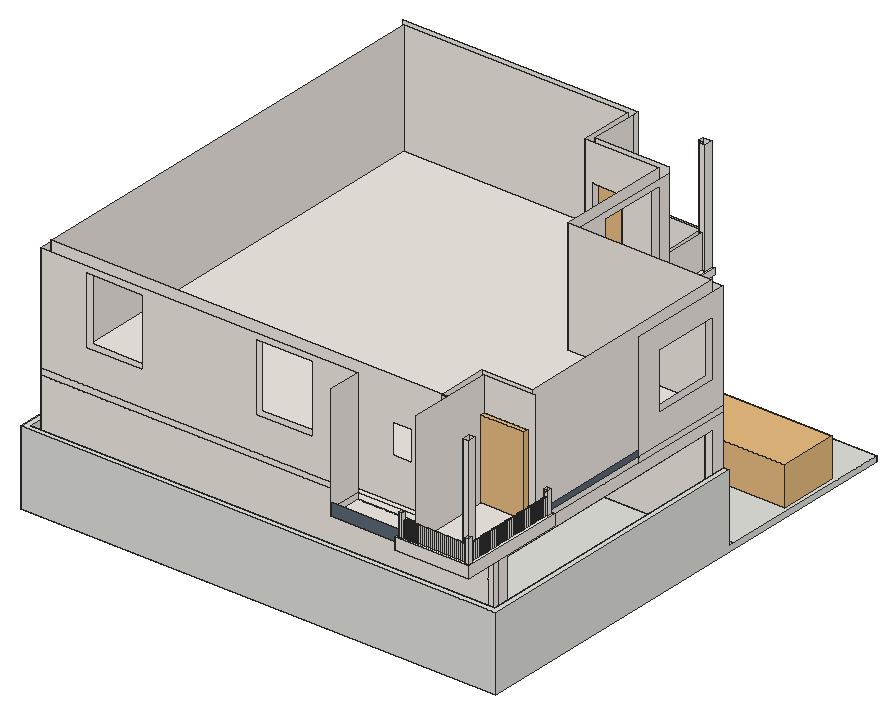
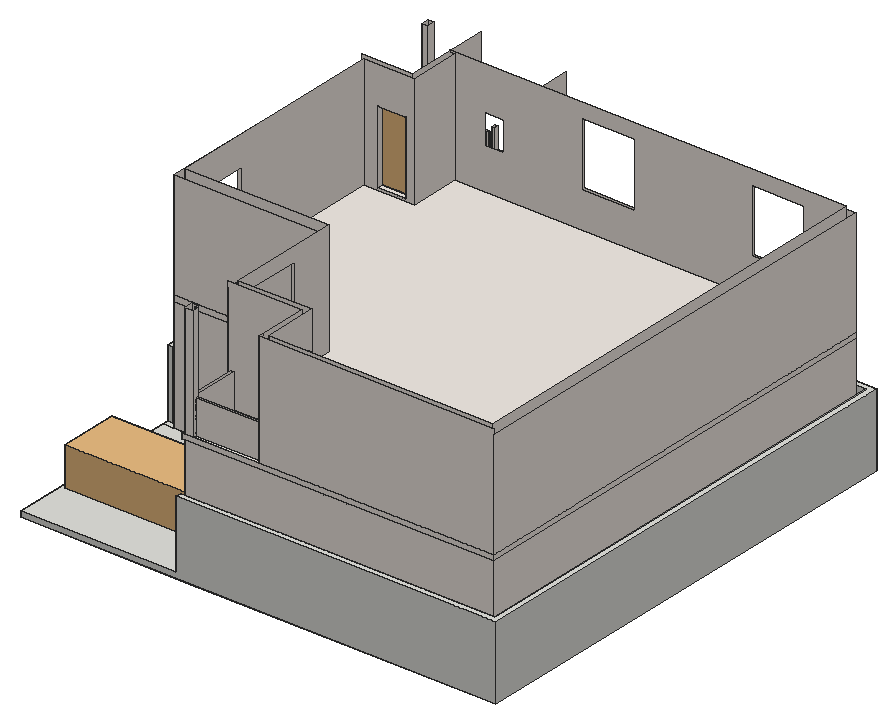
# SketchUp Ruby script. Lengths in inches.
U = 1.inch
M = Sketchup.active_model
def pt(a) = Geom::Point3d.new(a.map { |v| v * U })
def face(e, loops, mat)
  f = e.add_face(loops[0].map { |a| pt(a) })
  loops[1..].each { |l| e.add_face(l.map { |a| pt(a) }).erase! }
  f.material = f.back_material = mat if mat
  f
end
# faces: each face lists its corners as indices into pts; further lists are holes
def faces(e, pts, list, mat = nil) = list.each { |f| face(e, (f[0].is_a?(Array) ? f : [f]).map { |l| l.map { |i| pts[i] } }, mat) }
# xy, xz, yz: faces in a plane at the given z, y or x. An outline is a flat list of corners, or four numbers for a rectangle; further outlines are holes
def ring(l) = l.size == 4 ? [[l[0], l[1]], [l[2], l[1]], [l[2], l[3]], [l[0], l[3]]] : l.each_slice(2).to_a
def flat(e, list, mat, &to3) = list.each { |f| face(e, (f[0].is_a?(Array) ? f : [f]).map { |l| ring(l).map { |u, v| to3.(u, v) } }, mat) }
def xy(e, z, list, mat = nil) = flat(e, list, mat) { |x, y| [x, y, z] }
def xz(e, y, list, mat = nil) = flat(e, list, mat) { |x, z| [x, y, z] }
def yz(e, x, list, mat = nil) = flat(e, list, mat) { |y, z| [x, y, z] }
def lines(e, pts, list) = list.each { |a, b| e.add_line(pt(pts[a]), pt(pts[b])) }
# prism: a flat outline (further loops are holes) pulled along v
def prism(e, loops, v, mat = nil)
  f = face(e, loops, mat); d = Geom::Vector3d.new(v.map { |x| x * U })
  f.pushpull(f.normal.samedirection?(d) ? d.length : -d.length)
end
def box(e, o, s, mat = nil) = prism(e, [[o, [o[0] + s[0], o[1], o[2]], [o[0] + s[0], o[1] + s[1], o[2]], [o[0], o[1] + s[1], o[2]]]], [0, 0, s[2]], mat)
def at(x, y, z, deg = 0) = Geom::Transformation.translation(pt([x, y, z])) * Geom::Transformation.rotation(ORIGIN, Z_AXIS, deg.degrees)
def axes(o, x, y, z) = Geom::Transformation.new([*x, 0, *y, 0, *z, 0, *pt(o).to_a, 1])
def part(name) = M.definitions.add(name)
# library, detail: a bought-in or finely detailed component or shape, given as its bounding box
def library(name, o, s) = part(name).tap { |d| box(d.entities, o, s) }
def detail(e, o, s) = box(e.add_group.entities, o, s)
def put(e, d, t, mat = nil) = e.add_instance(d, t).tap { |i| i.material = mat if mat }
def group(e, t, mat = nil) = e.add_group.tap { |g| g.transformation = t; g.material = mat if mat }.entities
root = M.entities
M.materials.add("D01_Frost_White").color = [242, 235, 229]
M.materials.add("Denim_03_1K").color = [93, 106, 119]
c1 = library("2016+Honda+Civic+LX+Sedan",[0.01,0.03,0.02],[16.17,34.46,10.62])
c2 = library("porta+4",[0.2,-5.42,1.33],[46.55,4.72,83.21])
xy(root,-6,[[0,42,0,546,339,546,339,357,504,357,504,42],[339,357,504,546]])
xy(root,0,[[6,48,498,48,498,351,333,351,333,540,6,540],[333,351,504,351,504,357,339,357,339,540,333,540],[339,357,504,546]])
xy(root,0,[[[12,54,12,534,339,534,339,357,492,357,492,345,483,345,483,351,339,351,339,63,483,63,483,72,492,72,492,54],[21,63,333,63,333,351,189,351,189,63,183,63,183,351,21,351,21,207,183,207,183,201,21,201],[21,357,333,525]]],"D01_Frost_White")
xy(root,72,[[0,42,504,42,504,351,498,351,498,48,6,48,6,540,339,540,339,546,0,546]])
xy(root,108,[[483,72,492,108],[483,108,483,207,339,207,339,213,483,213,483,246,492,246,492,108],[483,246,492,345]],"D01_Frost_White")
xy(root,120,[[426,6,426,18,438,18,438,54,492,54,492,120,504,120,504,6],[348,18,438,54],[12,54,183,63],[183,54,189,63],[189,54,333,63],
  [333,54,339,534],[339,54,483,63],[483,54,486,54,486,60,492,60,492,357,483,357],[486,54,492,60],[12,63,21,201],
  [21,63,183,201],[183,63,189,357],[189,63,333,351],[339,63,483,207],[12,201,183,207],
  [12,207,21,351],[21,207,183,351],[339,207,483,213],[339,213,483,351],[12,351,183,357],
  [189,351,333,357],[339,351,483,357],[12,357,21,525],[21,357,183,525],[183,357,189,525],
  [189,357,333,525],[339,357,341.99,534],[12,525,183,534],[183,525,189,534],[189,525,333,534]],"D01_Frost_White")
xy(root,126,[[[432,12,498,12,498,114,492,114,492,108,438,108,438,18,432,18],[486,21.03,492,29]],[486,21.03,492,29],[18,60,432,60,432,114,486,114,486,351,333,351,333,471,255,471,255,528,18,528],[339,357,341.99,534],[261,477,333,528],
  [336,477,339,525],[333,525,339,525,339,534,330,534,330,528,333,528],[261,531,330,534]],"D01_Frost_White")
xy(root,129,[[441,108,471,114],[264,471,294,477]],"D01_Frost_White")
xy(root,131.92,[[499.1,72.74,500.6,73.14],[499.1,75.24,500.6,75.64],[499.1,77.74,500.6,78.14],[499.1,80.25,500.6,80.65],[499.1,82.75,500.6,83.15]],"D01_Frost_White")
xy(root,131.96,[[499.1,87.76,500.6,88.16],[499.1,90.26,500.6,90.66],[499.1,92.77,500.6,93.17],[499.1,95.27,500.6,95.67],[499.1,97.77,500.6,98.17],
  [499.1,100.28,500.6,100.68]],"D01_Frost_White")
xy(root,131.97,[[499.1,65.22,500.6,65.625],[499.1,67.73,500.6,68.13]],"D01_Frost_White")
xy(root,131.98,[[443.46,9.55,443.86,11.05],[445.61,9.55,446.01,11.05],[447.76,9.55,448.16,11.05],[449.9,9.55,450.3,11.05],[452.05,9.55,452.45,11.05],
  [454.19,9.55,454.59,11.05],[456.34,9.55,456.74,11.05],[458.48,9.55,458.88,11.05],[460.63,9.55,461.03,11.05],[462.77,9.55,463.17,11.05],
  [464.92,9.55,465.32,11.05],[467.06,9.55,467.46,11.05],[469.21,9.55,469.61,11.05],[471.36,9.55,471.76,11.05],[473.5,9.55,473.9,11.05],
  [475.65,9.55,476.05,11.05],[477.79,9.55,478.19,11.05],[479.9375,9.55,480.34,11.05],[482.08,9.55,482.48,11.05],[484.23,9.55,484.63,11.05],
  [486.375,9.55,486.77,11.05]],"D01_Frost_White")
xy(root,132,[[[426,6,504,6,504,120,492,120,492,114,498,114,498,12,432,12,432,18,426,18],[498.04,8.05,498.04,12.05,502.04,12.05,502.04,113.6,498.04,113.6,498.04,117.6,502.04,117.6,502.04,8.05],[428,8,432,12],[497.1,9.55,497.5,11.05],[494.96,9.55,495.36,11.05],[492.8125,9.55,493.21,11.05],[490.67,9.55,491.07,11.05],[488.52,9.55,488.92,11.05],[441.32,9.55,441.72,11.05],[439.17,9.55,439.57,11.05],[437.03,9.55,437.43,11.05],[434.88,9.55,435.28,11.05],[432.74,9.55,433.14,11.05],[499.1,112.8,500.6,113.2],[499.1,110.29,500.6,110.69],[499.1,107.79,500.6,108.1875],[499.1,105.28,500.6,105.68],[499.1,102.78,500.6,103.18],[499.1,85.25,500.6,85.65],[499.1,70.23,500.6,70.63],[499.1,62.72,500.6,63.12],[499.1,60.22,500.6,60.62],[499.1,57.71,500.6,58.11],[499.1,55.21,500.6,55.61],[499.1,52.71,500.6,53.11],[499.1,50.2,500.6,50.6],[499.1,47.7,500.6,48.1],[499.1,45.19,500.6,45.59],[499.1,42.69,500.6,43.09],[499.1,40.1875,500.6,40.59],[499.1,37.68,500.6,38.08],[499.1,35.18,500.6,35.58],[499.1,32.67,500.6,33.07],[499.1,30.17,500.6,30.57],[499.1,27.67,500.6,28.07],[499.1,25.16,500.6,25.5625],[499.1,22.66,500.6,23.06],[499.1,20.16,500.6,20.56],[499.1,17.65,500.6,18.05],[499.1,15.15,500.6,15.55],[499.1,12.64,500.6,13.04]]],"D01_Frost_White")
xz(root,6,[[426,120,504,132]],"D01_Frost_White")
xz(root,8,[[428,132,432,156]],"D01_Frost_White")
xz(root,8.05,[[498.04,132,502.04,156]],"D01_Frost_White")
xz(root,9.55,[[443.46,131.98,443.86,148.95],[445.61,131.98,446.01,148.95],[447.76,131.98,448.16,148.95],[449.9,131.98,450.3,148.95],[452.05,131.98,452.45,148.95],
  [454.19,131.98,454.59,148.95],[456.34,131.98,456.74,148.95],[458.48,131.98,458.88,148.95],[460.63,131.98,461.03,148.95],[462.77,131.98,463.17,148.95],
  [464.92,131.98,465.32,148.95],[467.06,131.98,467.46,148.95],[469.21,131.98,469.61,148.95],[471.36,131.98,471.76,148.95],[473.5,131.98,473.9,148.95],
  [475.65,131.98,476.05,148.95],[477.79,131.98,478.19,148.95],[479.9375,131.98,480.34,148.95],[482.08,131.98,482.48,148.95],[484.23,131.98,484.63,148.95],
  [486.375,131.98,486.77,148.95],[432.74,132,433.14,148.95],[434.88,132,435.28,148.95],[437.03,132,437.43,148.95],[439.17,132,439.57,148.95],
  [441.32,132,441.72,148.95],[488.52,132,488.92,148.95],[490.67,132,491.07,148.95],[492.8125,132,493.21,148.95],[494.96,132,495.36,148.95],
  [497.1,132,497.5,148.95]],"D01_Frost_White")
xz(root,11.05,[[443.46,131.98,443.86,148.95],[445.61,131.98,446.01,148.95],[447.76,131.98,448.16,148.95],[449.9,131.98,450.3,148.95],[452.05,131.98,452.45,148.95],
  [454.19,131.98,454.59,148.95],[456.34,131.98,456.74,148.95],[458.48,131.98,458.88,148.95],[460.63,131.98,461.03,148.95],[462.77,131.98,463.17,148.95],
  [464.92,131.98,465.32,148.95],[467.06,131.98,467.46,148.95],[469.21,131.98,469.61,148.95],[471.36,131.98,471.76,148.95],[473.5,131.98,473.9,148.95],
  [475.65,131.98,476.05,148.95],[477.79,131.98,478.19,148.95],[479.9375,131.98,480.34,148.95],[482.08,131.98,482.48,148.95],[484.23,131.98,484.63,148.95],
  [486.375,131.98,486.77,148.95],[432.74,132,433.14,148.95],[434.88,132,435.28,148.95],[437.03,132,437.43,148.95],[439.17,132,439.57,148.95],
  [441.32,132,441.72,148.95],[488.52,132,488.92,148.95],[490.67,132,491.07,148.95],[492.8125,132,493.21,148.95],[494.96,132,495.36,148.95],
  [497.1,132,497.5,148.95]],"D01_Frost_White")
xz(root,12,[[432,126,498,132],[428,132,432,156]],"D01_Frost_White")
xz(root,12.05,[[498.04,132,498.04,149.95,498.875,149.95,498.875,148.95,500.875,148.95,500.875,149.95,498.04,149.95,498.04,154.81,498.875,154.81,498.875,152.81,500.875,152.81,500.875,154.81,498.04,154.81,498.04,156,502.04,156,502.04,132]],"D01_Frost_White")
xz(root,12.64,[[499.1,132,500.6,148.95]],"D01_Frost_White")
xz(root,13.04,[[499.1,132,500.6,148.95]],"D01_Frost_White")
xz(root,15.15,[[499.1,132,500.6,148.95]],"D01_Frost_White")
xz(root,15.55,[[499.1,132,500.6,148.95]],"D01_Frost_White")
xz(root,17.65,[[499.1,132,500.6,148.95]],"D01_Frost_White")
xz(root,18,[[348,120,426,120,426,132,432,132,432,126,438,126,438,132.6,348,132.6]],"Denim_03_1K")
xz(root,18.05,[[499.1,132,500.6,148.95]],"D01_Frost_White")
xz(root,20.16,[[499.1,132,500.6,148.95]],"D01_Frost_White")
xz(root,20.56,[[499.1,132,500.6,148.95]],"D01_Frost_White")
xz(root,21.03,[[486,126,492,240]],"D01_Frost_White")
xz(root,22.66,[[499.1,132,500.6,148.95]],"D01_Frost_White")
xz(root,23.06,[[499.1,132,500.6,148.95]],"D01_Frost_White")
xz(root,25.16,[[499.1,132,500.6,148.95]],"D01_Frost_White")
xz(root,25.5625,[[499.1,132,500.6,148.95]],"D01_Frost_White")
xz(root,27.67,[[499.1,132,500.6,148.95]],"D01_Frost_White")
xz(root,28.07,[[499.1,132,500.6,148.95]],"D01_Frost_White")
xz(root,29,[[486,126,492,240]],"D01_Frost_White")
xz(root,30.17,[[499.1,132,500.6,148.95]],"D01_Frost_White")
xz(root,30.57,[[499.1,132,500.6,148.95]],"D01_Frost_White")
xz(root,32.67,[[499.1,132,500.6,148.95]],"D01_Frost_White")
xz(root,33.07,[[499.1,132,500.6,148.95]],"D01_Frost_White")
xz(root,35.18,[[499.1,132,500.6,148.95]],"D01_Frost_White")
xz(root,35.58,[[499.1,132,500.6,148.95]],"D01_Frost_White")
xz(root,37.68,[[499.1,132,500.6,148.95]],"D01_Frost_White")
xz(root,38.08,[[499.1,132,500.6,148.95]],"D01_Frost_White")
xz(root,40.1875,[[499.1,132,500.6,148.95]],"D01_Frost_White")
xz(root,40.59,[[499.1,132,500.6,148.95]],"D01_Frost_White")
xz(root,42,[[0,-6,504,72]])
xz(root,42.69,[[499.1,132,500.6,148.95]],"D01_Frost_White")
xz(root,43.09,[[499.1,132,500.6,148.95]],"D01_Frost_White")
xz(root,45.19,[[499.1,132,500.6,148.95]],"D01_Frost_White")
xz(root,45.59,[[499.1,132,500.6,148.95]],"D01_Frost_White")
xz(root,47.7,[[499.1,132,500.6,148.95]],"D01_Frost_White")
xz(root,48,[[6,0,498,72]])
xz(root,48.1,[[499.1,132,500.6,148.95]],"D01_Frost_White")
xz(root,50.2,[[499.1,132,500.6,148.95]],"D01_Frost_White")
xz(root,50.6,[[499.1,132,500.6,148.95]],"D01_Frost_White")
xz(root,52.71,[[499.1,132,500.6,148.95]],"D01_Frost_White")
xz(root,53.11,[[499.1,132,500.6,148.95]],"D01_Frost_White")
xz(root,54,[[12,0,486,120],[486,0,492,120],[12,120,348,126],[[12,126,348,240],[60,162,120,234],[240,162,300,234]]],"D01_Frost_White")
xz(root,55.21,[[499.1,132,500.6,148.95]],"D01_Frost_White")
xz(root,55.61,[[499.1,132,500.6,148.95]],"D01_Frost_White")
xz(root,57.71,[[499.1,132,500.6,148.95]],"D01_Frost_White")
xz(root,58.11,[[499.1,132,500.6,148.95]],"D01_Frost_White")
xz(root,60,[[[18,126,18,247.18,438,247.18,438,246,432,246,432,126],[62,164,118,232],[242,164,298,232],[380,170,400,202]]],"D01_Frost_White")
xz(root,60.22,[[499.1,132,500.6,148.95]],"D01_Frost_White")
xz(root,60.62,[[499.1,132,500.6,148.95]],"D01_Frost_White")
xz(root,62.72,[[499.1,132,500.6,148.95]],"D01_Frost_White")
xz(root,63,[[21,0,183,120],[183,0,189,120],[189,0,333,120],[339,0,339,120,483,120,483,108,461.45,108,461.45,0],[461.45,0,483,108]],"D01_Frost_White")
xz(root,63.12,[[499.1,132,500.6,148.95]],"D01_Frost_White")
xz(root,65.22,[[499.1,131.97,500.6,148.95]],"D01_Frost_White")
xz(root,65.625,[[499.1,131.97,500.6,148.95]],"D01_Frost_White")
xz(root,67.73,[[499.1,131.97,500.6,148.95]],"D01_Frost_White")
xz(root,68.13,[[499.1,131.97,500.6,148.95]],"D01_Frost_White")
xz(root,70.23,[[499.1,132,500.6,148.95]],"D01_Frost_White")
xz(root,70.63,[[499.1,132,500.6,148.95]],"D01_Frost_White")
xz(root,72,[[483,0,492,108]],"D01_Frost_White")
xz(root,72.74,[[499.1,131.92,500.6,148.95]],"D01_Frost_White")
xz(root,73.14,[[499.1,131.92,500.6,148.95]],"D01_Frost_White")
xz(root,75.24,[[499.1,131.92,500.6,148.95]],"D01_Frost_White")
xz(root,75.64,[[499.1,131.92,500.6,148.95]],"D01_Frost_White")
xz(root,77.74,[[499.1,131.92,500.6,148.95]],"D01_Frost_White")
xz(root,78.14,[[499.1,131.92,500.6,148.95]],"D01_Frost_White")
xz(root,80.25,[[499.1,131.92,500.6,148.95]],"D01_Frost_White")
xz(root,80.65,[[499.1,131.92,500.6,148.95]],"D01_Frost_White")
xz(root,82.75,[[499.1,131.92,500.6,148.95]],"D01_Frost_White")
xz(root,83.15,[[499.1,131.92,500.6,148.95]],"D01_Frost_White")
xz(root,85.25,[[499.1,132,500.6,148.95]],"D01_Frost_White")
xz(root,85.65,[[499.1,132,500.6,148.95]],"D01_Frost_White")
xz(root,87.76,[[499.1,131.96,500.6,148.95]],"D01_Frost_White")
xz(root,88.16,[[499.1,131.96,500.6,148.95]],"D01_Frost_White")
xz(root,90.26,[[499.1,131.96,500.6,148.95]],"D01_Frost_White")
xz(root,90.66,[[499.1,131.96,500.6,148.95]],"D01_Frost_White")
xz(root,92.77,[[499.1,131.96,500.6,148.95]],"D01_Frost_White")
xz(root,93.17,[[499.1,131.96,500.6,148.95]],"D01_Frost_White")
xz(root,95.27,[[499.1,131.96,500.6,148.95]],"D01_Frost_White")
xz(root,95.67,[[499.1,131.96,500.6,148.95]],"D01_Frost_White")
xz(root,97.77,[[499.1,131.96,500.6,148.95]],"D01_Frost_White")
xz(root,98.17,[[499.1,131.96,500.6,148.95]],"D01_Frost_White")
xz(root,100.28,[[499.1,131.96,500.6,148.95]],"D01_Frost_White")
xz(root,100.68,[[499.1,131.96,500.6,148.95]],"D01_Frost_White")
xz(root,102.78,[[499.1,132,500.6,148.95]],"D01_Frost_White")
xz(root,103.18,[[499.1,132,500.6,148.95]],"D01_Frost_White")
xz(root,105.28,[[499.1,132,500.6,148.95]],"D01_Frost_White")
xz(root,105.68,[[499.1,132,500.6,148.95]],"D01_Frost_White")
xz(root,107.79,[[499.1,132,500.6,148.95]],"D01_Frost_White")
xz(root,108,[[474,126,492,126,492,246,438,246,438,210,474,210],[[438,126,474,210],[441,129,471,207]]],"D01_Frost_White")
xz(root,108.1875,[[499.1,132,500.6,148.95]],"D01_Frost_White")
xz(root,110.29,[[499.1,132,500.6,148.95]],"D01_Frost_White")
xz(root,110.69,[[499.1,132,500.6,148.95]],"D01_Frost_White")
xz(root,112.8,[[499.1,132,500.6,148.95]],"D01_Frost_White")
xz(root,113.2,[[499.1,132,500.6,148.95]],"D01_Frost_White")
xz(root,113.6,[[[498.04,132,502.04,156],[498.875,147.95,498.875,154.81,500.875,154.81,500.875,152.81,498.875,152.81,498.875,149.95,500.875,149.95,500.875,147.95]]],"D01_Frost_White")
xz(root,114,[[[432,126,486,246],[441,129,471,207]],[492,126,498,132]],"D01_Frost_White")
xz(root,117.6,[[498.04,132,502.04,156]],"D01_Frost_White")
xz(root,120,[[492,120,504,132]],"D01_Frost_White")
xz(root,201,[[21,0,183,120]],"D01_Frost_White")
xz(root,207,[[21,0,183,120],[339,108,483,120]],"D01_Frost_White")
xz(root,213,[[339,108,483,120]],"D01_Frost_White")
xz(root,345,[[483,0,492,108]],"D01_Frost_White")
xz(root,351,[[498,0,504,72]])
xz(root,351,[[21,0,183,120],[189,0,333,120],[339,0,483,120],[333,126,486,246]],"D01_Frost_White")
xz(root,357,[[21,0,333,120],[339,0,492,120],[341.99,120,492,126],[339,126,492,240]],"D01_Frost_White")
xz(root,471,[[[255,126,333,246],[264,129,294,207]]],"D01_Frost_White")
xz(root,477,[[297,126,297,210,261,210,261,246,339,246,339,126,336,126,336,162,333,162,333,126],[[261,126,297,210],[264,129,294,207]]],"D01_Frost_White")
xz(root,525,[[21,0,333,120],[333,126,336,162],[336,126,339,126,339,246,333,246,333,162,336,162]],"D01_Frost_White")
xz(root,528,[[18,126,255,246],[261,126,330,162],[330,126,333,246]],"D01_Frost_White")
xz(root,531,[[261,126,330,162]],"D01_Frost_White")
xz(root,534,[[12,0,339,120],[12,120,341.99,126],[12,126,261,246],[330,126,339,246]],"D01_Frost_White")
xz(root,540,[[6,0,333,72],[333,0,339,72]])
xz(root,546,[[0,-6,0,72,339,72,339,0,504,0,504,-6]])
yz(root,0,[[42,-6,546,72]])
yz(root,6,[[48,0,540,72]])
yz(root,12,[[54,0,534,120],[54,120,534,126],[54,126,534,240]],"D01_Frost_White")
yz(root,18,[[60,126,528,246]],"D01_Frost_White")
yz(root,21,[[63,0,201,120],[207,0,351,120],[357,0,525,120]],"D01_Frost_White")
yz(root,183,[[63,0,201,120],[201,0,207,120],[207,0,351,120]],"D01_Frost_White")
yz(root,189,[[63,0,351,120]],"D01_Frost_White")
yz(root,255,[[471,126,528,246]],"D01_Frost_White")
yz(root,261,[[477,126,528,246],[531,126,534,126,534,246,528,246,528,162,531,162]],"D01_Frost_White")
yz(root,264,[[471,129,477,207]],"D01_Frost_White")
yz(root,294,[[471,129,477,207]],"D01_Frost_White")
yz(root,330,[[528,126,531,162],[531,126,531,162,528,162,528,246,534,246,534,126]],"D01_Frost_White")
yz(root,333,[[63,0,351,120],[357,0,525,120],[[351,126,471,246],[396,165,462,231]],[477,126,525,162],[525,126,528,246]],"D01_Frost_White")
yz(root,336,[[477,126,525,162]],"D01_Frost_White")
yz(root,339,[[540,0,546,72]])
yz(root,339,[[63,0,207,120],[207,0,213,108],[213,0,351,120],[357,0,534,120],[[357,126,477,240],[393,162,465,234]],
  [525,126,534,246]],"D01_Frost_White")
yz(root,341.99,[[357,120,534,126]],"D01_Frost_White")
yz(root,348,[[18,120,54,126],[18,126,54,240]],"D01_Frost_White")
yz(root,426,[[6,120,18,132]],"D01_Frost_White")
yz(root,428,[[8,132,12,156]],"D01_Frost_White")
yz(root,432,[[12,126,18,132],[60,126,114,246],[[8,132,12,156],[9.26,152.81,11.26,154.81],[9.26,148.95,11.26,149.95]]],"D01_Frost_White")
yz(root,432.74,[[9.55,132,11.05,148.95]],"D01_Frost_White")
yz(root,433.14,[[9.55,132,11.05,148.95]],"D01_Frost_White")
yz(root,434.88,[[9.55,132,11.05,148.95]],"D01_Frost_White")
yz(root,435.28,[[9.55,132,11.05,148.95]],"D01_Frost_White")
yz(root,437.03,[[9.55,132,11.05,148.95]],"D01_Frost_White")
yz(root,437.43,[[9.55,132,11.05,148.95]],"D01_Frost_White")
yz(root,438,[[18,126,108,246]],"D01_Frost_White")
yz(root,439.17,[[9.55,132,11.05,148.95]],"D01_Frost_White")
yz(root,439.57,[[9.55,132,11.05,148.95]],"D01_Frost_White")
yz(root,441,[[108,129,114,207]],"D01_Frost_White")
yz(root,441.32,[[9.55,132,11.05,148.95]],"D01_Frost_White")
yz(root,441.72,[[9.55,132,11.05,148.95]],"D01_Frost_White")
yz(root,443.46,[[9.55,131.98,11.05,148.95]],"D01_Frost_White")
yz(root,443.86,[[9.55,131.98,11.05,148.95]],"D01_Frost_White")
yz(root,445.61,[[9.55,131.98,11.05,148.95]],"D01_Frost_White")
yz(root,446.01,[[9.55,131.98,11.05,148.95]],"D01_Frost_White")
yz(root,447.76,[[9.55,131.98,11.05,148.95]],"D01_Frost_White")
yz(root,448.16,[[9.55,131.98,11.05,148.95]],"D01_Frost_White")
yz(root,449.9,[[9.55,131.98,11.05,148.95]],"D01_Frost_White")
yz(root,450.3,[[9.55,131.98,11.05,148.95]],"D01_Frost_White")
yz(root,452.05,[[9.55,131.98,11.05,148.95]],"D01_Frost_White")
yz(root,452.45,[[9.55,131.98,11.05,148.95]],"D01_Frost_White")
yz(root,454.19,[[9.55,131.98,11.05,148.95]],"D01_Frost_White")
yz(root,454.59,[[9.55,131.98,11.05,148.95]],"D01_Frost_White")
yz(root,456.34,[[9.55,131.98,11.05,148.95]],"D01_Frost_White")
yz(root,456.74,[[9.55,131.98,11.05,148.95]],"D01_Frost_White")
yz(root,458.48,[[9.55,131.98,11.05,148.95]],"D01_Frost_White")
yz(root,458.88,[[9.55,131.98,11.05,148.95]],"D01_Frost_White")
yz(root,460.63,[[9.55,131.98,11.05,148.95]],"D01_Frost_White")
yz(root,461.03,[[9.55,131.98,11.05,148.95]],"D01_Frost_White")
yz(root,462.77,[[9.55,131.98,11.05,148.95]],"D01_Frost_White")
yz(root,463.17,[[9.55,131.98,11.05,148.95]],"D01_Frost_White")
yz(root,464.92,[[9.55,131.98,11.05,148.95]],"D01_Frost_White")
yz(root,465.32,[[9.55,131.98,11.05,148.95]],"D01_Frost_White")
yz(root,467.06,[[9.55,131.98,11.05,148.95]],"D01_Frost_White")
yz(root,467.46,[[9.55,131.98,11.05,148.95]],"D01_Frost_White")
yz(root,469.21,[[9.55,131.98,11.05,148.95]],"D01_Frost_White")
yz(root,469.61,[[9.55,131.98,11.05,148.95]],"D01_Frost_White")
yz(root,471,[[108,129,114,207]],"D01_Frost_White")
yz(root,471.36,[[9.55,131.98,11.05,148.95]],"D01_Frost_White")
yz(root,471.76,[[9.55,131.98,11.05,148.95]],"D01_Frost_White")
yz(root,473.5,[[9.55,131.98,11.05,148.95]],"D01_Frost_White")
yz(root,473.9,[[9.55,131.98,11.05,148.95]],"D01_Frost_White")
yz(root,475.65,[[9.55,131.98,11.05,148.95]],"D01_Frost_White")
yz(root,476.05,[[9.55,131.98,11.05,148.95]],"D01_Frost_White")
yz(root,477.79,[[9.55,131.98,11.05,148.95]],"D01_Frost_White")
yz(root,478.19,[[9.55,131.98,11.05,148.95]],"D01_Frost_White")
yz(root,479.9375,[[9.55,131.98,11.05,148.95]],"D01_Frost_White")
yz(root,480.34,[[9.55,131.98,11.05,148.95]],"D01_Frost_White")
yz(root,482.08,[[9.55,131.98,11.05,148.95]],"D01_Frost_White")
yz(root,482.48,[[9.55,131.98,11.05,148.95]],"D01_Frost_White")
yz(root,483,[[63,0,72,108],[345,0,345,108,213,108,213,120,351,120,351,0],[63,108,111,120],[111,108,117,120],[117,108,135,120],
  [135,108,207,120]],"D01_Frost_White")
yz(root,484.23,[[9.55,131.98,11.05,148.95]],"D01_Frost_White")
yz(root,484.63,[[9.55,131.98,11.05,148.95]],"D01_Frost_White")
yz(root,486,[[54,120,60,126],[21.03,126,29,240],[[114,126,351,246],[275,158,343,214]]],"D01_Frost_White")
yz(root,486.375,[[9.55,131.98,11.05,148.95]],"D01_Frost_White")
yz(root,486.77,[[9.55,131.98,11.05,148.95]],"D01_Frost_White")
yz(root,488.52,[[9.55,132,11.05,148.95]],"D01_Frost_White")
yz(root,488.92,[[9.55,132,11.05,148.95]],"D01_Frost_White")
yz(root,490.67,[[9.55,132,11.05,148.95]],"D01_Frost_White")
yz(root,491.07,[[9.55,132,11.05,148.95]],"D01_Frost_White")
yz(root,492,[[54,0,60,120],[60,0,72,0,72,108,345,108,345,0,357,0,357,120,60,120],[120,120,246,126],[246,120,357,126],[21.03,126,29,240],
  [[246,126,357,240],[273,156,345,216]]],"D01_Frost_White")
yz(root,492,[[108,126,114,126,114,132,120,132,120,126,246,126,246,132.6,108,132.6]],"Denim_03_1K")
yz(root,492.8125,[[9.55,132,11.05,148.95]],"D01_Frost_White")
yz(root,493.21,[[9.55,132,11.05,148.95]],"D01_Frost_White")
yz(root,494.96,[[9.55,132,11.05,148.95]],"D01_Frost_White")
yz(root,495.36,[[9.55,132,11.05,148.95]],"D01_Frost_White")
yz(root,497.1,[[9.55,132,11.05,148.95]],"D01_Frost_White")
yz(root,497.5,[[9.55,132,11.05,148.95]],"D01_Frost_White")
yz(root,498,[[48,0,351,72]])
yz(root,498,[[12,126,114,132]],"D01_Frost_White")
yz(root,498.04,[[8.05,132,8.05,156,12.05,156,12.05,154.81,9.26,154.81,9.26,152.81,11.26,152.81,11.26,149.95,9.26,149.95,9.26,147.95,11.26,147.95,11.26,154.81,12.05,154.81,12.05,132],[113.6,132,117.6,156]],"D01_Frost_White")
yz(root,499.1,[[72.74,131.92,73.14,148.95],[75.24,131.92,75.64,148.95],[77.74,131.92,78.14,148.95],[80.25,131.92,80.65,148.95],[82.75,131.92,83.15,148.95],
  [87.76,131.96,88.16,148.95],[90.26,131.96,90.66,148.95],[92.77,131.96,93.17,148.95],[95.27,131.96,95.67,148.95],[97.77,131.96,98.17,148.95],
  [100.28,131.96,100.68,148.95],[65.22,131.97,65.625,148.95],[67.73,131.97,68.13,148.95],[12.64,132,13.04,148.95],[15.15,132,15.55,148.95],
  [17.65,132,18.05,148.95],[20.16,132,20.56,148.95],[22.66,132,23.06,148.95],[25.16,132,25.5625,148.95],[27.67,132,28.07,148.95],
  [30.17,132,30.57,148.95],[32.67,132,33.07,148.95],[35.18,132,35.58,148.95],[37.68,132,38.08,148.95],[40.1875,132,40.59,148.95],
  [42.69,132,43.09,148.95],[45.19,132,45.59,148.95],[47.7,132,48.1,148.95],[50.2,132,50.6,148.95],[52.71,132,53.11,148.95],
  [55.21,132,55.61,148.95],[57.71,132,58.11,148.95],[60.22,132,60.62,148.95],[62.72,132,63.12,148.95],[70.23,132,70.63,148.95],
  [85.25,132,85.65,148.95],[102.78,132,103.18,148.95],[105.28,132,105.68,148.95],[107.79,132,108.1875,148.95],[110.29,132,110.69,148.95],
  [112.8,132,113.2,148.95]],"D01_Frost_White")
yz(root,500.6,[[72.74,131.92,73.14,148.95],[75.24,131.92,75.64,148.95],[77.74,131.92,78.14,148.95],[80.25,131.92,80.65,148.95],[82.75,131.92,83.15,148.95],
  [87.76,131.96,88.16,148.95],[90.26,131.96,90.66,148.95],[92.77,131.96,93.17,148.95],[95.27,131.96,95.67,148.95],[97.77,131.96,98.17,148.95],
  [100.28,131.96,100.68,148.95],[65.22,131.97,65.625,148.95],[67.73,131.97,68.13,148.95],[12.64,132,13.04,148.95],[15.15,132,15.55,148.95],
  [17.65,132,18.05,148.95],[20.16,132,20.56,148.95],[22.66,132,23.06,148.95],[25.16,132,25.5625,148.95],[27.67,132,28.07,148.95],
  [30.17,132,30.57,148.95],[32.67,132,33.07,148.95],[35.18,132,35.58,148.95],[37.68,132,38.08,148.95],[40.1875,132,40.59,148.95],
  [42.69,132,43.09,148.95],[45.19,132,45.59,148.95],[47.7,132,48.1,148.95],[50.2,132,50.6,148.95],[52.71,132,53.11,148.95],
  [55.21,132,55.61,148.95],[57.71,132,58.11,148.95],[60.22,132,60.62,148.95],[62.72,132,63.12,148.95],[70.23,132,70.63,148.95],
  [85.25,132,85.65,148.95],[102.78,132,103.18,148.95],[105.28,132,105.68,148.95],[107.79,132,108.1875,148.95],[110.29,132,110.69,148.95],
  [112.8,132,113.2,148.95]],"D01_Frost_White")
yz(root,502.04,[[8.05,132,12.05,156],[113.6,132,117.6,156]],"D01_Frost_White")
yz(root,504,[[42,-6,546,-6,546,0,351,0,351,72,42,72]])
yz(root,504,[[6,120,120,132]],"D01_Frost_White")
p = [[339,357,0],[339,357,-6],[486,54,126],[486,29,126]]
lines(root,p,[[0,1],[2,3]])
put(root,c1,axes([367.65,492.17,-0.09],[0,-3.841,0],[3.841,0,0],[0,0,3.841]))
put(root,c2,at(437.8,108.7,125.46))
put(root,c2,at(250.25,482.42,125.46))
